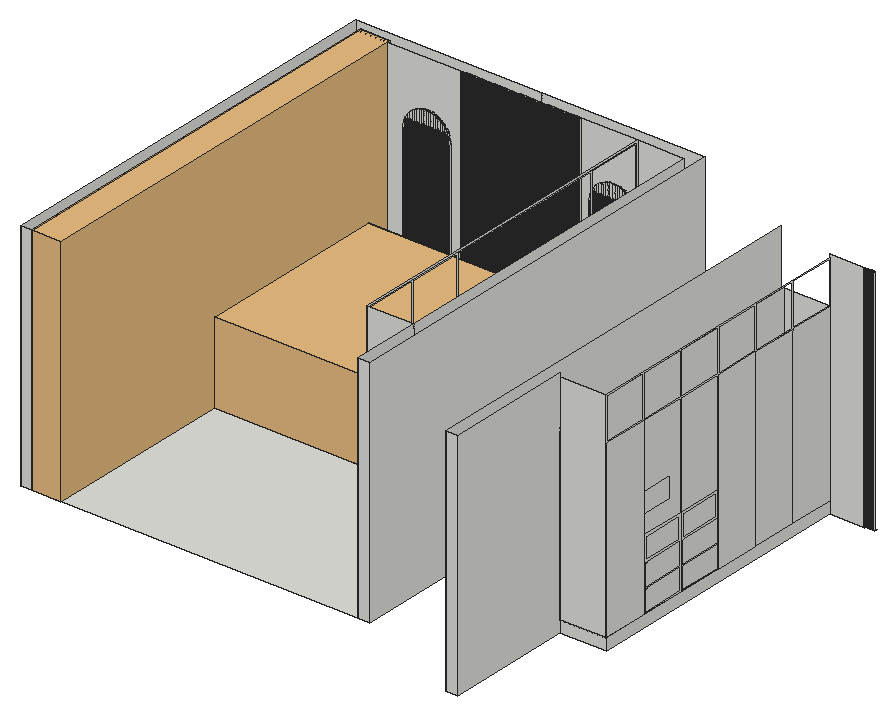
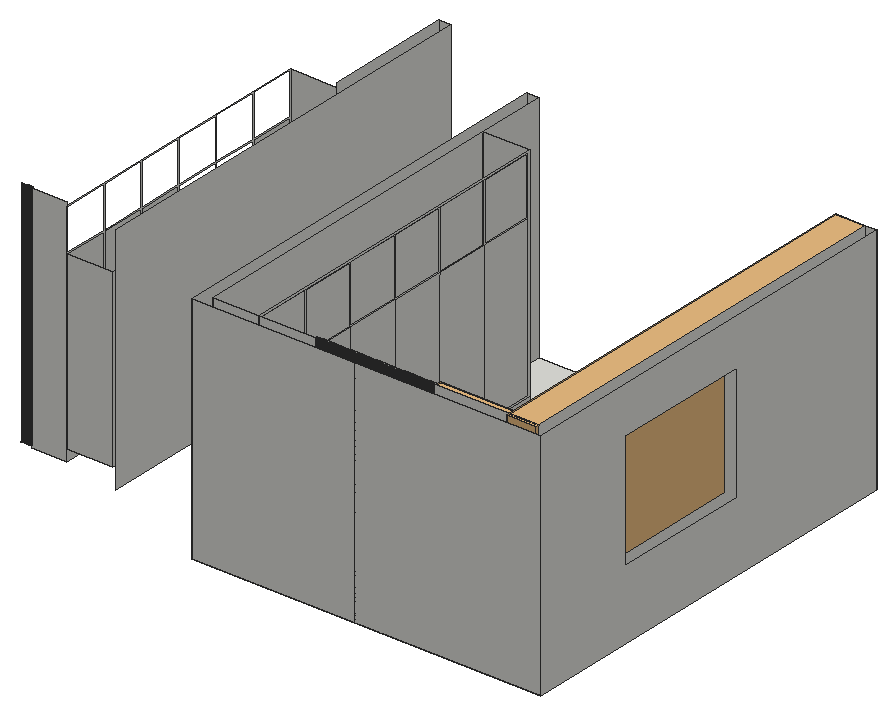
# SketchUp Ruby script. Lengths in inches.
U = 1.inch
M = Sketchup.active_model
def pt(a) = Geom::Point3d.new(a.map { |v| v * U })
def face(e, loops, mat)
  f = e.add_face(loops[0].map { |a| pt(a) })
  loops[1..].each { |l| e.add_face(l.map { |a| pt(a) }).erase! }
  f.material = f.back_material = mat if mat
  f
end
# faces: each face lists its corners as indices into pts; further lists are holes
def faces(e, pts, list, mat = nil) = list.each { |f| face(e, (f[0].is_a?(Array) ? f : [f]).map { |l| l.map { |i| pts[i] } }, mat) }
# xy, xz, yz: faces in a plane at the given z, y or x. An outline is a flat list of corners, or four numbers for a rectangle; further outlines are holes
def ring(l) = l.size == 4 ? [[l[0], l[1]], [l[2], l[1]], [l[2], l[3]], [l[0], l[3]]] : l.each_slice(2).to_a
def flat(e, list, mat, &to3) = list.each { |f| face(e, (f[0].is_a?(Array) ? f : [f]).map { |l| ring(l).map { |u, v| to3.(u, v) } }, mat) }
def xy(e, z, list, mat = nil) = flat(e, list, mat) { |x, y| [x, y, z] }
def xz(e, y, list, mat = nil) = flat(e, list, mat) { |x, z| [x, y, z] }
def yz(e, x, list, mat = nil) = flat(e, list, mat) { |y, z| [x, y, z] }
def lines(e, pts, list) = list.each { |a, b| e.add_line(pt(pts[a]), pt(pts[b])) }
# prism: a flat outline (further loops are holes) pulled along v
def prism(e, loops, v, mat = nil)
  f = face(e, loops, mat); d = Geom::Vector3d.new(v.map { |x| x * U })
  f.pushpull(f.normal.samedirection?(d) ? d.length : -d.length)
end
def box(e, o, s, mat = nil) = prism(e, [[o, [o[0] + s[0], o[1], o[2]], [o[0] + s[0], o[1] + s[1], o[2]], [o[0], o[1] + s[1], o[2]]]], [0, 0, s[2]], mat)
def at(x, y, z, deg = 0) = Geom::Transformation.translation(pt([x, y, z])) * Geom::Transformation.rotation(ORIGIN, Z_AXIS, deg.degrees)
def axes(o, x, y, z) = Geom::Transformation.new([*x, 0, *y, 0, *z, 0, *pt(o).to_a, 1])
def part(name) = M.definitions.add(name)
# library, detail: a bought-in or finely detailed component or shape, given as its bounding box
def library(name, o, s) = part(name).tap { |d| box(d.entities, o, s) }
def detail(e, o, s) = box(e.add_group.entities, o, s)
def put(e, d, t, mat = nil) = e.add_instance(d, t).tap { |i| i.material = mat if mat }
def group(e, t, mat = nil) = e.add_group.tap { |g| g.transformation = t; g.material = mat if mat }.entities
root = M.entities
c1 = library("Curtains with rod",[2.65,-2.46,0.02],[153.34,15.02,114.15])
c2 = part("Headboard wall slat")
box(c2.entities,[0,-1,0],[1,1,120])
c3 = library("Platform bed",[0,0,0],[83.59,112.46,35.43])
xy(root,0,[[0,24.57,0,240.57,180,240.57,180,24.57,174,24.57,174,234.57,6,234.57,6,24.57],[6,24.57,174,24.57,174,60.57,150,60.57,150,233.57,148.8,233.57,148.8,234.57,148.6,234.57,148.6,233.57,147.6,233.57,147.6,234.57,147.4,234.57,147.4,233.57,146.4,233.57,146.4,234.57,146.2,234.57,146.2,233.57,145.2,233.57,145.2,234.57,145,234.57,145,233.57,144,233.57,144,234.57,143.8,234.57,143.8,233.57,142.8,233.57,142.8,234.57,142.6,234.57,142.6,233.57,141.6,233.57,141.6,234.57,141.4,234.57,141.4,233.57,140.4,233.57,140.4,234.57,140.2,234.57,140.2,233.57,139.2,233.57,139.2,234.57,139,234.57,139,233.57,138,233.57,138,234.57,137.8,234.57,137.8,233.57,136.8,233.57,136.8,234.57,136.6,234.57,136.6,233.57,135.6,233.57,135.6,234.57,135.4,234.57,135.4,233.57,134.4,233.57,134.4,234.57,134.2,234.57,134.2,233.57,133.2,233.57,133.2,234.57,133,234.57,133,233.57,132,233.57,132,234.57,131.8,234.57,131.8,233.57,130.8,233.57,130.8,234.57,130.6,234.57,130.6,233.57,129.6,233.57,129.6,234.57,129.4,234.57,129.4,233.57,128.4,233.57,128.4,234.57,128.2,234.57,128.2,233.57,127.2,233.57,127.2,234.57,127,234.57,127,233.57,126,233.57,126,234.57,54,234.57,54,233.69,52.8,233.69,52.8,234.57,52.6,234.57,52.6,233.69,51.6,233.69,51.6,234.57,51.4,234.57,51.4,233.69,50.4,233.69,50.4,234.57,50.2,234.57,50.2,233.57,49.2,233.57,49.2,234.57,49,234.57,49,233.57,48,233.57,48,234.57,47.8,234.57,47.8,233.57,46.8,233.57,46.8,234.57,46.6,234.57,46.6,233.57,45.6,233.57,45.6,234.57,45.4,234.57,45.4,233.57,44.4,233.57,44.4,234.57,44.2,234.57,44.2,233.57,43.2,233.57,43.2,234.57,43,234.57,43,233.57,42,233.57,42,234.57,41.8,234.57,41.8,233.57,40.8,233.57,40.8,234.57,40.6,234.57,40.6,233.57,39.6,233.57,39.6,234.57,39.4,234.57,39.4,233.57,38.4,233.57,38.4,234.57,38.2,234.57,38.2,233.57,37.2,233.57,37.2,234.57,37,234.57,37,233.57,36,233.57,36,234.57,35.8,234.57,35.8,233.57,34.8,233.57,34.8,234.57,34.6,234.57,34.6,233.57,33.6,233.57,33.6,234.57,33.4,234.57,33.4,233.57,32.4,233.57,32.4,234.57,32.2,234.57,32.2,233.57,31.2,233.57,31.2,234.57,31,234.57,31,233.57,30,233.57,30,234.57,6,234.57],[30,233.57,31,234.57],[31.2,233.57,32.2,234.57],[32.4,233.57,33.4,234.57],
  [33.6,233.57,34.6,234.57],[34.8,233.57,35.8,234.57],[36,233.57,37,234.57],[37.2,233.57,38.2,234.57],[38.4,233.57,39.4,234.57],
  [39.6,233.57,40.6,234.57],[40.8,233.57,41.8,234.57],[42,233.57,43,234.57],[43.2,233.57,44.2,234.57],[44.4,233.57,45.4,234.57],
  [45.6,233.57,46.6,234.57],[46.8,233.57,47.8,234.57],[48,233.57,49,234.57],[49.2,233.57,50.2,234.57],[126,233.57,127,234.57],
  [127.2,233.57,128.2,234.57],[128.4,233.57,129.4,234.57],[129.6,233.57,130.6,234.57],[130.8,233.57,131.8,234.57],[132,233.57,133,234.57],
  [133.2,233.57,134.2,234.57],[134.4,233.57,135.4,234.57],[135.6,233.57,136.6,234.57],[136.8,233.57,137.8,234.57],[138,233.57,139,234.57],
  [139.2,233.57,140.2,234.57],[140.4,233.57,141.4,234.57],[141.6,233.57,142.6,234.57],[142.8,233.57,143.8,234.57],[144,233.57,145,234.57],
  [145.2,233.57,146.2,234.57],[146.4,233.57,147.4,234.57],[147.6,233.57,148.6,234.57],[148.8,233.57,149.8,234.57],[149.8,233.57,150,234.57],
  [50.4,233.69,51.4,234.57],[51.6,233.69,52.6,234.57],[52.8,233.69,54,234.57]])
xy(root,1,[[287,209,288,210],[288.2,209,289.2,210],[289.4,209,290.4,210],[290.6,209,291.6,210],[291.8,209,292.8,210]])
xy(root,6,[[245,66,268.82,210],[268.82,66,269,210]])
xy(root,6.2,[[268.82,66.2,269,89.8],[268.82,138.2,269,161.8],[268.82,162.2,269,185.8],[268.82,186.2,269,209.8]])
xy(root,7,[[150,61.57,150.18,233.57]])
xy(root,7.01,[[268.82,91.2,269,112.76],[268.82,115.2,269,136.8]])
xy(root,7.2,[[150,61.77,150.18,89.2],[150,89.6,150.18,118.04],[150,118.4375,150.18,146.87],[150,147.27,150.18,175.7],[150,176.1,150.18,204.54],
  [150,204.9375,150.18,233.37]])
xy(root,17.7,[[268.82,91.2,269,112.76],[268.82,115.2,269,136.8]])
xy(root,18.7,[[268.82,91.2,269,112.8],[268.82,115.2,269,136.8]])
xy(root,29.7,[[268.82,91.2,269,112.8],[268.82,115.2,269,136.8]])
xz(root,0,[[239,0,245,120]])
xz(root,24.57,[[0,0,6,120],[174,0,180,120]])
xz(root,60.57,[[150,0,174,120]])
xz(root,61.57,[[150,7,150.18,119]])
xz(root,61.77,[[150,7.2,150.18,88.8]])
xz(root,66,[[245,0,269,6],[245,6,268.82,118]])
xz(root,66.2,[[268.82,6.2,269,95.8]])
xz(root,89.2,[[150,7.2,150.18,88.8]])
xz(root,89.6,[[150,7.2,150.18,88.8]])
xz(root,89.8,[[268.82,6.2,269,95.8]])
xz(root,91.2,[[268.82,7.01,269,17.7],[268.82,18.7,269,29.7]])
xz(root,112.76,[[268.82,7.01,269,17.7]])
xz(root,112.8,[[268.82,18.7,269,29.7]])
xz(root,115.2,[[268.82,7.01,269,17.7],[268.82,18.7,269,29.7]])
xz(root,118.04,[[150,7.2,150.18,88.8]])
xz(root,118.4375,[[150,7.2,150.18,88.8]])
xz(root,136.8,[[268.82,7.01,269,17.7],[268.82,18.7,269,29.7]])
xz(root,138.2,[[268.82,6.2,269,95.8]])
xz(root,146.87,[[150,7.2,150.18,88.8]])
xz(root,147.27,[[150,7.2,150.18,88.8]])
xz(root,161.8,[[268.82,6.2,269,95.8]])
xz(root,162.2,[[268.82,6.2,269,95.8]])
xz(root,175.7,[[150,7.2,150.18,88.8]])
xz(root,176.1,[[150,7.2,150.18,88.8]])
xz(root,185.8,[[268.82,6.2,269,95.8]])
xz(root,186.2,[[268.82,6.2,269,95.8]])
xz(root,204.54,[[150,7.2,150.18,88.8]])
xz(root,204.9375,[[150,7.2,150.18,88.8]])
xz(root,209,[[287,1,288,120],[288.2,1,289.2,120],[289.4,1,290.4,120],[290.6,1,291.6,120],[291.8,1,292.8,120]])
xz(root,209.8,[[268.82,6.2,269,95.8]])
xz(root,210,[[269,0,287,0,287,120,269,120,269,118,268.82,118,268.82,6,269,6],[287,1,288,120],[288,1,288.2,120],[288.2,1,289.2,120],[289.2,1,289.4,120],
  [289.4,1,290.4,120],[290.4,1,290.6,120],[290.6,1,291.6,120],[291.6,1,291.8,120],[245,6,268.82,96]])
xz(root,233.37,[[150,7.2,150.18,84]])
xz(root,233.57,[[30,0,31,0,31,88.79,30.91,88.59,30.8,88.3,30.6875,88.01,30.59,87.71,30.49,87.41,30.41,87.11,30.33,86.8,30.26,86.49,30.2,86.1875,30.15,85.88,30.1,85.57,30.07,85.25,30.04,84.94,30.02,84.63,30,84.3125],[31.2,0,32.2,0,32.2,90.92,32.11,90.8,31.9375,90.54,31.77,90.27,31.45,89.73,31.2,89.23],[32.4,0,33.4,0,33.4,92.37,33.3,92.26,33.08,92.03,32.67,91.55,32.48,91.31,32.4,91.2],[33.6,0,34.6,0,34.6,93.45,34.45,93.33,33.97,92.92,33.74,92.7,33.6,92.57],[34.8,0,35.8,0,35.8,94.27,35.73,94.23,35.46,94.0625,35.2,93.89,34.95,93.71,34.8,93.6],
  [36,0,37,0,37,94.91,36.83,94.83,36.27,94.55,36,94.39],[37.2,0,38.2,0,38.2,95.38,37.99,95.3125,37.7,95.2,37.41,95.09,37.2,95],[38.4,0,39.4,0,39.4,95.71,39.2,95.67,38.89,95.59,38.59,95.51,38.4,95.45],[39.6,0,40.6,0,40.6,95.92,40.43,95.9,40.12,95.85,39.8125,95.8,39.6,95.76],[40.8,0,41.8,0,41.8,96,41.6875,96,41.37,95.98,41.06,95.96,40.75,95.93,40.8,89.23],
  [42,0,43,0,43,95.96,42.94,95.96,42.63,95.98,42.6,95.98,42.3125,96,42,96],[43.2,0,44.2,0,44.2,88.79,44.1875,95.8,43.88,95.85,43.57,95.9,43.25,95.93,43.2,95.9375],[44.4,0,45.4,0,45.4,88.79,45.41,95.51,45.11,95.59,44.8,95.67,44.49,95.74,44.39,95.76,44.4,89.23],[45.6,0,46.6,0,46.6,88.79,46.59,95.09,46.3,95.2,46.01,95.3125,45.71,95.41,45.6,95.45],[46.8,0,47.8,0,47.8,88.79,47.73,94.55,47.17,94.83,46.88,94.96,46.79,95,46.8,89.23],
  [48,0,49,0,49,88.79,49.05,93.71,48.8,93.89,48.54,94.0625,48.27,94.23,48,94.39],[49.2,0,50.2,0,50.2,92.76,50.03,92.92,49.55,93.33,49.31,93.52,49.2,89.23],[126,0,127,0,127,88.53,126.41,87.11,126,84],[127.2,0,128.2,0,128.2,90.77,127.61,90,127.2,89.02],[128.4,0,129.4,0,129.4,92.34,128.4,91.03],
  [129.6,0,130.6,0,130.6,93.32,129.6,92.55],[130.8,0,131.8,0,131.8,94.27,131.73,94.23,131.46,94.0625,131.2,93.89,130.95,93.71,130.8,93.6],[132,0,133,0,133,94.91,132.83,94.83,132.27,94.55,132,94.39],[133.2,0,134.2,0,134.2,95.38,133.99,95.3125,133.7,95.2,133.41,95.09,133.2,95],[134.4,0,135.4,0,135.4,95.71,135.2,95.67,134.89,95.59,134.59,95.51,134.4,95.45],
  [135.6,0,136.6,0,136.6,95.92,136.43,95.9,136.12,95.85,135.8125,95.8,135.6,95.76],[136.8,0,137.8,0,137.8,96,137.6875,96,137.37,95.98,137.06,95.96,136.75,95.93,136.8,89.23],[138,0,139,0,139,95.96,138.94,95.96,138.63,95.98,138.6,95.98,138.3125,96,138,96],[139.2,0,140.2,0,140.2,88.79,140.1875,95.8,139.88,95.85,139.57,95.9,139.25,95.93,139.2,95.9375],[140.4,0,141.4,0,141.4,88.79,141.41,95.51,141.11,95.59,140.8,95.67,140.49,95.74,140.39,95.76,140.4,89.23],
  [141.6,0,142.6,0,142.6,88.79,142.59,95.09,142.3,95.2,142.01,95.3125,141.71,95.41,141.6,95.45],[142.8,0,143.8,0,143.8,88.79,143.73,94.55,143.17,94.83,142.88,94.96,142.79,95,142.8,89.23],[144,0,145,0,145,88.79,145.05,93.71,144.8,93.89,144.54,94.0625,144.27,94.23,144,94.39],[145.2,0,146.2,0,146.2,92.76,146.03,92.92,145.55,93.33,145.31,93.52,145.2,89.23],[146.4,0,147.4,0,147.4,91.46,147.33,91.55,146.92,92.03,146.7,92.26,146.49,92.49,146.4,92.57],
  [147.6,0,148.6,0,148.6,89.62,148.55,89.73,148.23,90.27,148.0625,90.54,147.89,90.8,147.71,91.05,147.6,91.2],[148.8,0,150,0,150,84.3125,149.98,84.63,149.96,84.94,149.93,85.25,149.9,85.57,149.85,85.88,149.8,86.1875,149.74,86.49,149.67,86.8,149.59,87.11,149.51,87.41,149.41,87.71,149.3125,88.01,149.2,88.3,149.09,88.59,148.83,89.17,148.8,89.23],[150,7,150.18,84]])
xz(root,233.69,[[50.4,0,51.4,0,51.4,91.46,51.33,91.55,50.92,92.03,50.7,92.26,50.49,92.49,50.4,92.57],[51.6,0,52.6,0,52.6,89.62,52.55,89.73,52.23,90.27,52.0625,90.54,51.89,90.8,51.71,91.05,51.6,91.2],[52.8,0,54,0,54,84.3125,53.98,84.63,53.96,84.94,53.93,85.25,53.9,85.57,53.85,85.88,53.8,86.1875,53.74,86.49,53.67,86.8,53.59,87.11,53.51,87.41,53.41,87.71,53.3125,88.01,53.2,88.3,53.09,88.59,52.83,89.17,52.8,89.23]])
xz(root,234.57,[[6,0,30,0,30,84.3125,30.02,84.63,30.04,84.94,30.07,85.25,30.1,85.57,30.15,85.88,30.2,86.1875,30.26,86.49,30.33,86.8,30.41,87.11,30.49,87.41,30.59,87.71,30.6875,88.01,30.8,88.3,30.91,88.59,31,88.79,31.04,88.88,31.17,89.17,31.45,89.73,31.77,90.27,31.9375,90.54,32.11,90.8,32.2,90.92,32.29,91.05,32.4,91.2,32.48,91.31,32.67,91.55,33.08,92.03,33.3,92.26,33.4,92.37,33.51,92.49,33.6,92.57,33.74,92.7,33.97,92.92,34.45,93.33,34.6,93.45,34.69,93.52,34.8,93.6,34.95,93.71,35.2,93.89,35.46,94.0625,35.73,94.23,35.8,94.27,36,94.39,36.27,94.55,36.83,94.83,37,94.91,37.12,94.96,37.2,95,37.41,95.09,37.7,95.2,37.99,95.3125,38.2,95.38,38.29,95.41,38.4,95.45,38.59,95.51,38.89,95.59,39.2,95.67,39.4,95.71,39.51,95.74,39.6,95.76,39.8125,95.8,40.12,95.85,40.43,95.9,40.6,95.92,40.75,95.93,41.06,95.96,41.37,95.98,41.6875,96,42.3125,96,42.6,95.98,42.63,95.98,42.94,95.96,43,95.96,43.2,95.9375,43.25,95.93,43.57,95.9,43.88,95.85,44.1875,95.8,44.39,95.76,44.49,95.74,44.8,95.67,45.11,95.59,45.41,95.51,45.6,95.45,45.71,95.41,46.01,95.3125,46.3,95.2,46.59,95.09,46.79,95,46.88,94.96,47.17,94.83,47.73,94.55,48.27,94.23,48.54,94.0625,48.8,93.89,49.05,93.71,49.31,93.52,49.55,93.33,50.03,92.92,50.2,92.76,50.26,92.7,50.4,92.57,50.49,92.49,50.7,92.26,50.92,92.03,51.33,91.55,51.4,91.46,51.52,91.31,51.6,91.2,51.71,91.05,51.89,90.8,52.0625,90.54,52.23,90.27,52.55,89.73,52.6,89.62,52.69,89.45,52.83,89.17,53.09,88.59,53.2,88.3,53.3125,88.01,53.41,87.71,53.51,87.41,53.59,87.11,53.67,86.8,53.74,86.49,53.8,86.1875,53.85,85.88,53.9,85.57,53.93,85.25,53.96,84.94,53.98,84.63,54,84.3125,54,0,60,0,60,120,6,120],[30,0,31,0,31,88.79,30.91,88.59,30.8,88.3,30.6875,88.01,30.59,87.71,30.49,87.41,30.41,87.11,30.33,86.8,30.26,86.49,30.2,86.1875,30.15,85.88,30.1,85.57,30.07,85.25,30.04,84.94,30.02,84.63,30,84.3125],[31,0,31.2,0,31.2,89.23,31.17,89.17,31.04,88.88,31,88.79],[31.2,0,32.2,0,32.2,90.92,32.11,90.8,31.9375,90.54,31.77,90.27,31.45,89.73,31.2,89.23],[32.2,0,32.4,0,32.4,91.2,32.29,91.05,32.2,90.92],
  [32.4,0,33.4,0,33.4,92.37,33.3,92.26,33.08,92.03,32.67,91.55,32.48,91.31,32.4,91.2],[33.4,0,33.6,0,33.6,92.57,33.51,92.49,33.4,92.37],[33.6,0,34.6,0,34.6,93.45,34.45,93.33,33.97,92.92,33.74,92.7,33.6,92.57],[34.6,0,34.8,0,34.8,93.6,34.69,93.52,34.6,93.45],[34.8,0,35.8,0,35.8,94.27,35.73,94.23,35.46,94.0625,35.2,93.89,34.95,93.71,34.8,93.6],
  [35.8,0,36,0,36,94.39,35.8,94.27],[36,0,37,0,37,94.91,36.83,94.83,36.27,94.55,36,94.39],[37,0,37.2,0,37.2,95,37.12,94.96,37,94.91],[37.2,0,38.2,0,38.2,95.38,37.99,95.3125,37.7,95.2,37.41,95.09,37.2,95],[38.2,0,38.4,0,38.4,95.45,38.29,95.41,38.2,95.38],
  [38.4,0,39.4,0,39.4,95.71,39.2,95.67,38.89,95.59,38.59,95.51,38.4,95.45],[39.4,0,39.6,0,39.6,95.76,39.51,95.74,39.4,95.71],[39.6,0,40.6,0,40.6,95.92,40.43,95.9,40.12,95.85,39.8125,95.8,39.6,95.76],[40.6,0,40.8,0,40.8,89.23,40.75,95.93,40.6,95.92],[40.8,0,41.8,0,41.8,96,41.6875,96,41.37,95.98,41.06,95.96,40.75,95.93,40.8,89.23],
  [41.8,0,42,96],[42,0,43,0,43,95.96,42.94,95.96,42.63,95.98,42.6,95.98,42.3125,96,42,96],[43,0,43.2,0,43.2,95.9375,43,95.96],[43.2,0,44.2,0,44.2,88.79,44.1875,95.8,43.88,95.85,43.57,95.9,43.25,95.93,43.2,95.9375],[44.2,0,44.4,0,44.4,89.23,44.39,95.76,44.1875,95.8,44.2,88.79],
  [44.4,0,45.4,0,45.4,88.79,45.41,95.51,45.11,95.59,44.8,95.67,44.49,95.74,44.39,95.76,44.4,89.23],[45.4,0,45.6,0,45.6,95.45,45.41,95.51,45.4,88.79],[45.6,0,46.6,0,46.6,88.79,46.59,95.09,46.3,95.2,46.01,95.3125,45.71,95.41,45.6,95.45],[46.6,0,46.8,0,46.8,89.23,46.79,95,46.59,95.09,46.6,88.79],[46.8,0,47.8,0,47.8,88.79,47.73,94.55,47.17,94.83,46.88,94.96,46.79,95,46.8,89.23],
  [47.8,0,48,0,48,94.39,47.73,94.55,47.8,88.79],[48,0,49,0,49,88.79,49.05,93.71,48.8,93.89,48.54,94.0625,48.27,94.23,48,94.39],[49,0,49.2,0,49.2,89.23,49.31,93.52,49.05,93.71,49,88.79],[49.2,0,50.2,0,50.2,92.76,50.03,92.92,49.55,93.33,49.31,93.52,49.2,89.23],[50.2,0,50.4,0,50.4,92.57,50.26,92.7,50.2,92.76],
  [50.4,0,51.4,0,51.4,91.46,51.33,91.55,50.92,92.03,50.7,92.26,50.49,92.49,50.4,92.57],[51.4,0,51.6,0,51.6,91.2,51.52,91.31,51.4,91.46],[51.6,0,52.6,0,52.6,89.62,52.55,89.73,52.23,90.27,52.0625,90.54,51.89,90.8,51.71,91.05,51.6,91.2],[52.6,0,52.8,0,52.8,89.23,52.69,89.45,52.6,89.62],[52.8,0,54,0,54,84.3125,53.98,84.63,53.96,84.94,53.93,85.25,53.9,85.57,53.85,85.88,53.8,86.1875,53.74,86.49,53.67,86.8,53.59,87.11,53.51,87.41,53.41,87.71,53.3125,88.01,53.2,88.3,53.09,88.59,52.83,89.17,52.8,89.23],
  [60,0,61,120],[61,0,102,120],[102,0,120,120],[120,0,121,120],[121,0,126,0,126,84,126.41,87.11,127,88.53,127.2,89.02,127.61,90,128.2,90.77,128.4,91.03,129.4,92.34,129.51,92.49,129.6,92.55,130.6,93.32,130.8,93.47,130.8,93.6,130.95,93.71,131.2,93.89,131.46,94.0625,131.73,94.23,131.8,94.27,132,94.39,132.27,94.55,132.83,94.83,133,94.91,133.12,94.96,133.2,95,133.41,95.09,133.7,95.2,133.99,95.3125,134.2,95.38,134.29,95.41,134.4,95.45,134.59,95.51,134.89,95.59,135.2,95.67,135.4,95.71,135.51,95.74,135.6,95.76,135.8125,95.8,136.12,95.85,136.43,95.9,136.6,95.92,136.75,95.93,137.06,95.96,137.37,95.98,137.6875,96,138.3125,96,138.6,95.98,138.63,95.98,138.94,95.96,139,95.96,139.2,95.9375,139.25,95.93,139.57,95.9,139.88,95.85,140.1875,95.8,140.39,95.76,140.49,95.74,140.8,95.67,141.11,95.59,141.41,95.51,141.6,95.45,141.71,95.41,142.01,95.3125,142.3,95.2,142.59,95.09,142.79,95,142.88,94.96,143.17,94.83,143.73,94.55,144.27,94.23,144.54,94.0625,144.8,93.89,145.05,93.71,145.31,93.52,145.55,93.33,146.03,92.92,146.2,92.76,146.26,92.7,146.4,92.57,146.49,92.49,146.7,92.26,146.92,92.03,147.33,91.55,147.4,91.46,147.52,91.31,147.6,91.2,147.71,91.05,147.89,90.8,148.0625,90.54,148.23,90.27,148.55,89.73,148.6,89.62,148.69,89.45,148.83,89.17,149.09,88.59,149.2,88.3,149.3125,88.01,149.41,87.71,149.51,87.41,149.59,87.11,149.67,86.8,149.74,86.49,149.8,86.1875,149.85,85.88,149.9,85.57,149.93,85.25,149.96,84.94,149.98,84.63,150,84.3125,150,84,150,120,121,120],
  [126,0,127,0,127,88.53,126.41,87.11,126,84],[127,0,127.2,0,127.2,89.02,127,88.53],[127.2,0,128.2,0,128.2,90.77,127.61,90,127.2,89.02],[128.2,0,128.4,0,128.4,91.03,128.2,90.77],[128.4,0,129.4,0,129.4,92.34,128.4,91.03],
  [129.4,0,129.6,0,129.6,92.55,129.51,92.49,129.4,92.34],[129.4,0,129.6,0,129.6,92.57,129.51,92.49,129.4,92.37],[129.6,0,130.6,0,130.6,93.32,129.6,92.55],[130.6,0,130.8,0,130.8,93.47,130.6,93.32],[130.8,0,131.8,0,131.8,94.27,131.73,94.23,131.46,94.0625,131.2,93.89,130.95,93.71,130.8,93.6],
  [131.8,0,132,0,132,94.39,131.8,94.27],[132,0,133,0,133,94.91,132.83,94.83,132.27,94.55,132,94.39],[133,0,133.2,0,133.2,95,133.12,94.96,133,94.91],[133.2,0,134.2,0,134.2,95.38,133.99,95.3125,133.7,95.2,133.41,95.09,133.2,95],[134.2,0,134.4,0,134.4,95.45,134.29,95.41,134.2,95.38],
  [134.4,0,135.4,0,135.4,95.71,135.2,95.67,134.89,95.59,134.59,95.51,134.4,95.45],[135.4,0,135.6,0,135.6,95.76,135.51,95.74,135.4,95.71],[135.6,0,136.6,0,136.6,95.92,136.43,95.9,136.12,95.85,135.8125,95.8,135.6,95.76],[136.6,0,136.8,0,136.8,89.23,136.75,95.93,136.6,95.92],[136.8,0,137.8,0,137.8,96,137.6875,96,137.37,95.98,137.06,95.96,136.75,95.93,136.8,89.23],
  [137.8,0,138,96],[138,0,139,0,139,95.96,138.94,95.96,138.63,95.98,138.6,95.98,138.3125,96,138,96],[139,0,139.2,0,139.2,95.9375,139,95.96],[139.2,0,140.2,0,140.2,88.79,140.1875,95.8,139.88,95.85,139.57,95.9,139.25,95.93,139.2,95.9375],[140.2,0,140.4,0,140.4,89.23,140.39,95.76,140.1875,95.8,140.2,88.79],
  [140.4,0,141.4,0,141.4,88.79,141.41,95.51,141.11,95.59,140.8,95.67,140.49,95.74,140.39,95.76,140.4,89.23],[141.4,0,141.6,0,141.6,95.45,141.41,95.51,141.4,88.79],[141.6,0,142.6,0,142.6,88.79,142.59,95.09,142.3,95.2,142.01,95.3125,141.71,95.41,141.6,95.45],[142.6,0,142.8,0,142.8,89.23,142.79,95,142.59,95.09,142.6,88.79],[142.8,0,143.8,0,143.8,88.79,143.73,94.55,143.17,94.83,142.88,94.96,142.79,95,142.8,89.23],
  [143.8,0,144,0,144,94.39,143.73,94.55,143.8,88.79],[144,0,145,0,145,88.79,145.05,93.71,144.8,93.89,144.54,94.0625,144.27,94.23,144,94.39],[145,0,145.2,0,145.2,89.23,145.31,93.52,145.05,93.71,145,88.79],[145.2,0,146.2,0,146.2,92.76,146.03,92.92,145.55,93.33,145.31,93.52,145.2,89.23],[146.2,0,146.4,0,146.4,92.57,146.26,92.7,146.2,92.76],
  [146.4,0,147.4,0,147.4,91.46,147.33,91.55,146.92,92.03,146.7,92.26,146.49,92.49,146.4,92.57],[147.4,0,147.6,0,147.6,91.2,147.52,91.31,147.4,91.46],[147.6,0,148.6,0,148.6,89.62,148.55,89.73,148.23,90.27,148.0625,90.54,147.89,90.8,147.71,91.05,147.6,91.2],[148.6,0,148.8,0,148.8,89.23,148.69,89.45,148.6,89.62],[148.8,0,150,0,150,84.3125,149.98,84.63,149.96,84.94,149.93,85.25,149.9,85.57,149.85,85.88,149.8,86.1875,149.74,86.49,149.67,86.8,149.59,87.11,149.51,87.41,149.41,87.71,149.3125,88.01,149.2,88.3,149.09,88.59,148.83,89.17,148.8,89.23],
  [150,0,174,6],[150,6,174,120]])
xz(root,240.57,[[0,0,96,120],[96,0,180,120]])
yz(root,0,[[[24.57,0,240.57,120],[114.57,36,186.57,96]]])
yz(root,6,[[[24.57,0,234.57,120],[114.57,36,186.57,96]]])
yz(root,30,[[233.57,0,234.57,84]])
yz(root,31,[[233.57,0,234.57,88.79]])
yz(root,31.2,[[233.57,0,234.57,89.23]])
yz(root,32.2,[[233.57,0,234.57,88.79]])
yz(root,32.4,[[233.57,0,234.57,89.23]])
yz(root,33.4,[[233.57,0,234.57,88.79]])
yz(root,33.6,[[233.57,0,234.57,89.23]])
yz(root,34.6,[[233.57,0,234.57,88.79]])
yz(root,34.8,[[233.57,0,234.57,89.23]])
yz(root,35.8,[[233.57,0,234.57,88.79]])
yz(root,36,[[233.57,0,234.57,89.23]])
yz(root,37,[[233.57,0,234.57,88.79]])
yz(root,37.2,[[233.57,0,234.57,89.23]])
yz(root,38.2,[[233.57,0,234.57,88.79]])
yz(root,38.4,[[233.57,0,234.57,89.23]])
yz(root,39.4,[[233.57,0,234.57,88.79]])
yz(root,39.6,[[233.57,0,234.57,89.23]])
yz(root,40.6,[[233.57,0,234.57,88.79]])
yz(root,40.8,[[233.57,0,234.57,89.23]])
yz(root,41.8,[[233.57,0,234.57,88.79]])
yz(root,42,[[233.57,0,234.57,89.23]])
yz(root,43,[[233.57,0,234.57,0.1875],[233.57,0.1875,234.57,88.79]])
yz(root,43.2,[[233.57,0,234.57,89.23]])
yz(root,44.2,[[233.57,0,234.57,88.79]])
yz(root,44.4,[[233.57,0,234.57,89.23]])
yz(root,45.4,[[233.57,0,234.57,88.79]])
yz(root,45.6,[[233.57,0,234.57,89.23]])
yz(root,46.6,[[233.57,0,234.57,88.79]])
yz(root,46.8,[[233.57,0,234.57,89.23]])
yz(root,47.8,[[233.57,0,234.57,88.79]])
yz(root,48,[[233.57,0,234.57,89.23]])
yz(root,49,[[233.57,0,234.57,88.79]])
yz(root,49.2,[[233.57,0,234.57,89.23]])
yz(root,50.2,[[233.57,0,234.57,88.79]])
yz(root,50.4,[[233.69,0,234.57,89.23]])
yz(root,51.4,[[233.69,0,234.57,88.79]])
yz(root,51.6,[[233.69,0,234.57,89.23]])
yz(root,52.6,[[233.69,0,234.57,88.79]])
yz(root,52.8,[[233.69,0,234.57,89.23]])
yz(root,54,[[233.69,0,234.57,84]])
yz(root,126,[[233.57,0,234.57,84]])
yz(root,127,[[233.57,0,234.57,88.53]])
yz(root,127.2,[[233.57,0,234.57,89.02]])
yz(root,128.2,[[233.57,0,234.57,88.79]])
yz(root,128.4,[[233.57,0,234.57,89.23]])
yz(root,129.4,[[233.57,0,234.57,88.79]])
yz(root,129.6,[[233.57,0,234.57,89.23]])
yz(root,130.6,[[233.57,0,234.57,88.79]])
yz(root,130.8,[[233.57,0,234.57,89.23]])
yz(root,131.8,[[233.57,0,234.57,88.79]])
yz(root,132,[[233.57,0,234.57,89.23]])
yz(root,133,[[233.57,0,234.57,88.79]])
yz(root,133.2,[[233.57,0,234.57,89.23]])
yz(root,134.2,[[233.57,0,234.57,88.79]])
yz(root,134.4,[[233.57,0,234.57,89.23]])
yz(root,135.4,[[233.57,0,234.57,88.79]])
yz(root,135.6,[[233.57,0,234.57,89.23]])
yz(root,136.6,[[233.57,0,234.57,88.79]])
yz(root,136.8,[[233.57,0,234.57,89.23]])
yz(root,137.8,[[233.57,0,234.57,88.79]])
yz(root,138,[[233.57,0,234.57,89.23]])
yz(root,139,[[233.57,0,234.57,0.1875],[233.57,0.1875,234.57,88.79]])
yz(root,139.2,[[233.57,0,234.57,89.23]])
yz(root,140.2,[[233.57,0,234.57,88.79]])
yz(root,140.4,[[233.57,0,234.57,89.23]])
yz(root,141.4,[[233.57,0,234.57,88.79]])
yz(root,141.6,[[233.57,0,234.57,89.23]])
yz(root,142.6,[[233.57,0,234.57,88.79]])
yz(root,142.8,[[233.57,0,234.57,89.23]])
yz(root,143.8,[[233.57,0,234.57,88.79]])
yz(root,144,[[233.57,0,234.57,89.23]])
yz(root,145,[[233.57,0,234.57,88.79]])
yz(root,145.2,[[233.57,0,234.57,89.23]])
yz(root,146.2,[[233.57,0,234.57,88.79]])
yz(root,146.4,[[233.57,0,234.57,89.23]])
yz(root,147.4,[[233.57,0,234.57,88.79]])
yz(root,147.6,[[233.57,0,234.57,89.23]])
yz(root,148.6,[[233.57,0,234.57,88.79]])
yz(root,148.8,[[233.57,0,234.57,89.23]])
yz(root,150,[[60.57,0,233.57,6],[233.57,0,234.57,6],[60.57,6,60.57,120,234.57,120,234.57,84,233.57,84,233.57,119,61.57,119,61.57,7,233.57,7,233.57,6],[233.57,6,234.57,84],[61.77,7.2,89.2,88.8],
  [89.6,7.2,118.04,88.8],[118.4375,7.2,146.87,88.8],[147.27,7.2,175.7,88.8],[176.1,7.2,204.54,88.8],[204.9375,7.2,233.37,88.8]])
yz(root,150.18,[[[61.57,7,233.57,119],[147.27,7.2,175.7,88.8],[89.6,7.2,118.04,88.8],[118.4375,7.2,146.87,88.8],[176.1,7.2,204.54,88.8],[204.9375,7.2,233.37,88.8],[61.77,7.2,89.2,88.8],[147.27,89.2,175.7,118.8],[89.6,89.2,118.04,118.8],[204.9375,89.2,233.37,118.8],[176.1,89.2,204.54,118.8],[118.4375,89.2,146.87,118.8],[61.77,89.2,89.2,118.8]]])
yz(root,174,[[24.57,0,60.57,120],[60.57,0,234.57,6],[60.57,6,234.57,120]])
yz(root,180,[[24.57,0,240.57,120]])
yz(root,239,[[0,0,216,120]])
yz(root,245,[[0,0,66,120],[[66,6,210,96],[91.2,30.7,112.8,41.7],[115.2,30.7,136.8,41.7]]])
yz(root,268.82,[[[66,6,210,118],[90.2,6.2,113.8,95.8],[114.2,6.2,137.8,95.8],[186.2,6.2,209.8,95.8],[162.2,6.2,185.8,95.8],[138.2,6.2,161.8,95.8],[66.2,6.2,89.8,95.8],[90.2,96.2,113.8,117.8],[186.2,96.2,209.8,117.8],[162.2,96.2,185.8,117.8],[138.2,96.2,161.8,117.8],[66.2,96.2,89.8,117.8],[114.2,96.2,137.8,117.8]],[[90.2,6.2,113.8,42.7],[91.2,30.7,112.8,41.7],[91.2,18.7,112.8,29.7],[91.2,7.01,112.76,17.7]],[[114.2,6.2,137.8,42.7],[115.2,30.7,136.8,41.7],[115.2,18.7,136.8,29.7],[115.2,7.01,136.8,17.7]]])
yz(root,269,[[66,0,210,6],[66.2,6.2,89.8,95.8],[138.2,6.2,161.8,95.8],[162.2,6.2,185.8,95.8],[186.2,6.2,209.8,95.8],
  [91.2,7.01,112.76,17.7],[115.2,7.01,136.8,17.7],[91.2,18.7,112.8,29.7],[115.2,18.7,136.8,29.7]])
yz(root,287,[[209,1,210,120]])
yz(root,288,[[209,1,210,120]])
yz(root,288.2,[[209,1,210,120]])
yz(root,289.2,[[209,1,210,120]])
yz(root,289.4,[[209,1,210,120]])
yz(root,290.4,[[209,1,210,120]])
yz(root,290.6,[[209,1,210,120]])
yz(root,291.6,[[209,1,210,120]])
yz(root,291.8,[[209,1,210,120]])
put(root,c1,axes([18.56,20.9375,-0.02],[0,1.38,0],[-1,0,0],[0,0,1.0512]))
put(root,c2,at(60,234.57,0))
put(root,c2,at(61.2,234.57,0))
put(root,c2,at(62.4,234.57,0))
put(root,c2,at(63.6,234.57,0))
put(root,c2,at(64.8,234.57,0))
put(root,c2,at(66,234.57,0))
put(root,c2,at(67.2,234.57,0))
put(root,c2,at(68.4,234.57,0))
put(root,c2,at(69.6,234.57,0))
put(root,c2,at(70.8,234.57,0))
put(root,c2,at(72,234.57,0))
put(root,c2,at(73.2,234.57,0))
put(root,c2,at(74.4,234.57,0))
put(root,c2,at(75.6,234.57,0))
put(root,c2,at(76.8,234.57,0))
put(root,c2,at(78,234.57,0))
put(root,c3,axes([145.4,123.22,0],[0,1.18437,0],[-1.18437,0,0],[0,0,1.18437]))
put(root,c2,at(79.2,234.57,0))
put(root,c2,at(80.4,234.57,0))
put(root,c2,at(81.6,234.57,0))
put(root,c2,at(82.8,234.57,0))
put(root,c2,at(84,234.57,0))
put(root,c2,at(85.2,234.57,0))
put(root,c2,at(86.4,234.57,0))
put(root,c2,at(87.6,234.57,0))
put(root,c2,at(88.8,234.57,0))
put(root,c2,at(90,234.57,0))
put(root,c2,at(91.2,234.57,0))
put(root,c2,at(92.4,234.57,0))
put(root,c2,at(93.6,234.57,0))
put(root,c2,at(94.8,234.57,0))
put(root,c2,at(96,234.57,0))
put(root,c2,at(97.2,234.57,0))
put(root,c2,at(98.4,234.57,0))
put(root,c2,at(99.6,234.57,0))
put(root,c2,at(100.8,234.57,0))
put(root,c2,at(102,234.57,0))
put(root,c2,at(103.2,234.57,0))
put(root,c2,at(104.4,234.57,0))
put(root,c2,at(105.6,234.57,0))
put(root,c2,at(106.8,234.57,0))
put(root,c2,at(108,234.57,0))
put(root,c2,at(109.2,234.57,0))
put(root,c2,at(110.4,234.57,0))
put(root,c2,at(111.6,234.57,0))
put(root,c2,at(112.8,234.57,0))
put(root,c2,at(114,234.57,0))
put(root,c2,at(115.2,234.57,0))
put(root,c2,at(116.4,234.57,0))
put(root,c2,at(117.6,234.57,0))
put(root,c2,at(118.8,234.57,0))
put(root,c2,at(120,234.57,0))
